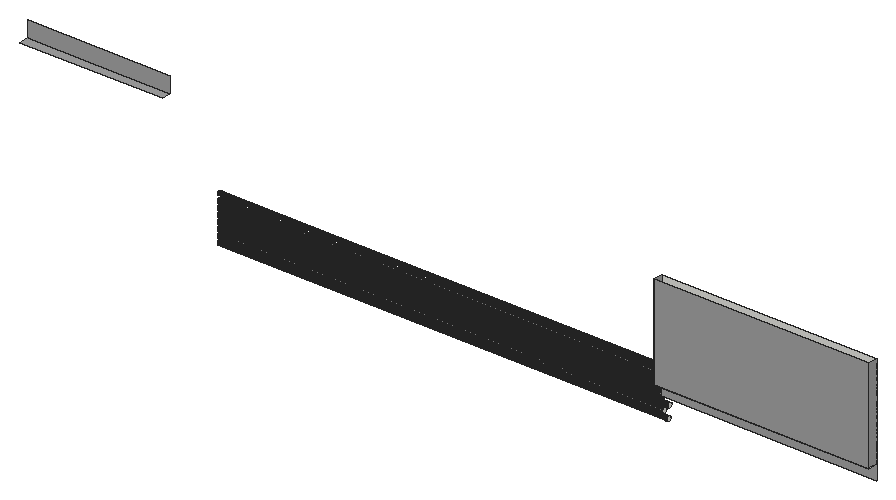
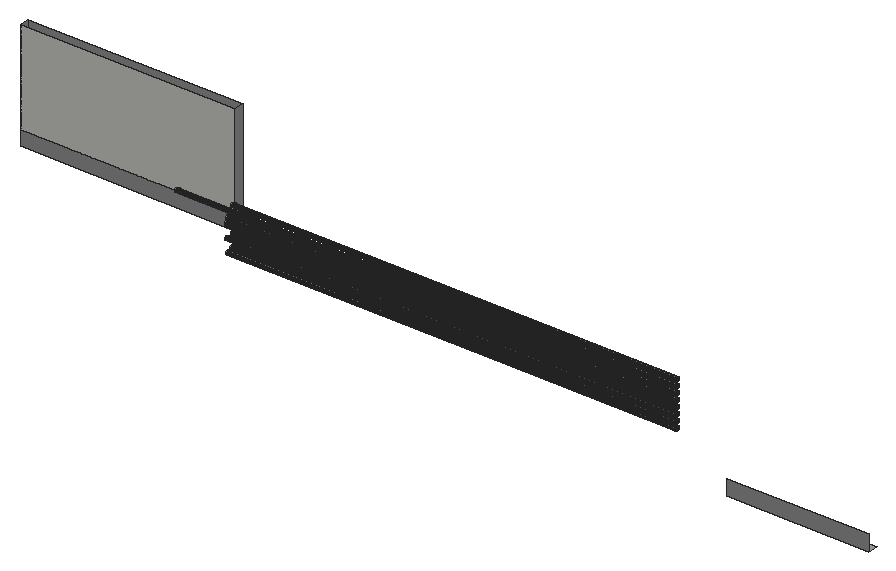
# SketchUp Ruby script. Lengths in inches.
U = 1.inch
M = Sketchup.active_model
def pt(a) = Geom::Point3d.new(a.map { |v| v * U })
def face(e, loops, mat)
  f = e.add_face(loops[0].map { |a| pt(a) })
  loops[1..].each { |l| e.add_face(l.map { |a| pt(a) }).erase! }
  f.material = f.back_material = mat if mat
  f
end
# faces: each face lists its corners as indices into pts; further lists are holes
def faces(e, pts, list, mat = nil) = list.each { |f| face(e, (f[0].is_a?(Array) ? f : [f]).map { |l| l.map { |i| pts[i] } }, mat) }
# xy, xz, yz: faces in a plane at the given z, y or x. An outline is a flat list of corners, or four numbers for a rectangle; further outlines are holes
def ring(l) = l.size == 4 ? [[l[0], l[1]], [l[2], l[1]], [l[2], l[3]], [l[0], l[3]]] : l.each_slice(2).to_a
def flat(e, list, mat, &to3) = list.each { |f| face(e, (f[0].is_a?(Array) ? f : [f]).map { |l| ring(l).map { |u, v| to3.(u, v) } }, mat) }
def xy(e, z, list, mat = nil) = flat(e, list, mat) { |x, y| [x, y, z] }
def xz(e, y, list, mat = nil) = flat(e, list, mat) { |x, z| [x, y, z] }
def yz(e, x, list, mat = nil) = flat(e, list, mat) { |y, z| [x, y, z] }
def lines(e, pts, list) = list.each { |a, b| e.add_line(pt(pts[a]), pt(pts[b])) }
# prism: a flat outline (further loops are holes) pulled along v
def prism(e, loops, v, mat = nil)
  f = face(e, loops, mat); d = Geom::Vector3d.new(v.map { |x| x * U })
  f.pushpull(f.normal.samedirection?(d) ? d.length : -d.length)
end
def box(e, o, s, mat = nil) = prism(e, [[o, [o[0] + s[0], o[1], o[2]], [o[0] + s[0], o[1] + s[1], o[2]], [o[0], o[1] + s[1], o[2]]]], [0, 0, s[2]], mat)
def at(x, y, z, deg = 0) = Geom::Transformation.translation(pt([x, y, z])) * Geom::Transformation.rotation(ORIGIN, Z_AXIS, deg.degrees)
def axes(o, x, y, z) = Geom::Transformation.new([*x, 0, *y, 0, *z, 0, *pt(o).to_a, 1])
def part(name) = M.definitions.add(name)
# library, detail: a bought-in or finely detailed component or shape, given as its bounding box
def library(name, o, s) = part(name).tap { |d| box(d.entities, o, s) }
def detail(e, o, s) = box(e.add_group.entities, o, s)
def put(e, d, t, mat = nil) = e.add_instance(d, t).tap { |i| i.material = mat if mat }
def group(e, t, mat = nil) = e.add_group.tap { |g| g.transformation = t; g.material = mat if mat }.entities
root = M.entities
M.materials.add("[0133_Gray]").color = [128, 128, 128]
M.materials.add("[Pavers Flagstone Gray]").color = [162, 162, 162]
xy(root,165.99,[[229.62,0,297.58,3]],"[Pavers Flagstone Gray]")
xy(root,166.5625,[[0,36,45.0625,39]],"[Pavers Flagstone Gray]")
xz(root,0,[[229.62,165.99,297.58,195.875]],"[Pavers Flagstone Gray]")
xz(root,3,[[229.62,165.99,297.58,195.875]])
xz(root,3,[[229.62,161.3125,297.58,165.99]],"[Pavers Flagstone Gray]")
xz(root,39,[[0,166.5625,45.0625,171.57]],"[Pavers Flagstone Gray]")
yz(root,229.62,[[4.01,168.41,4.17,168.43,4.32,168.49,4.45,168.59,4.55,168.72,4.61,168.87,4.63,169.03,4.61,169.19,4.55,169.34,4.45,169.47,4.32,169.57,4.17,169.64,4.01,169.66,3.84,169.64,3.69,169.57,3.5625,169.47,3.46,169.34,3.4,169.19,3.38,169.03,3.4,168.87,3.46,168.72,3.5625,168.59,3.69,168.49,3.84,168.43]])
yz(root,229.62,[[0,165.99,3,195.875]],"[Pavers Flagstone Gray]")
yz(root,229.78,[[4.01,156.41,4.17,156.43,4.32,156.49,4.45,156.59,4.55,156.72,4.61,156.87,4.63,157.03,4.61,157.19,4.55,157.34,4.45,157.47,4.32,157.57,4.17,157.64,4.01,157.66,3.84,157.64,3.69,157.57,3.5625,157.47,3.46,157.34,3.4,157.19,3.38,157.03,3.4,156.87,3.46,156.72,3.5625,156.59,3.69,156.49,3.84,156.43]])
yz(root,231.1,[[4.01,154.41,4.17,154.43,4.32,154.49,4.45,154.59,4.55,154.72,4.61,154.87,4.63,155.03,4.61,155.19,4.55,155.34,4.45,155.47,4.32,155.57,4.17,155.64,4.01,155.66,3.84,155.64,3.69,155.57,3.5625,155.47,3.46,155.34,3.4,155.19,3.38,155.03,3.4,154.87,3.46,154.72,3.5625,154.59,3.69,154.49,3.84,154.43],[4.01,164.41,4.17,164.43,4.32,164.49,4.45,164.59,4.55,164.72,4.61,164.87,4.63,165.03,4.61,165.19,4.55,165.34,4.45,165.47,4.32,165.57,4.17,165.64,4.01,165.66,3.84,165.64,3.69,165.57,3.5625,165.47,3.46,165.34,3.4,165.19,3.38,165.03,3.4,164.87,3.46,164.72,3.5625,164.59,3.69,164.49,3.84,164.43]])
yz(root,231.41,[[4.01,158.41,4.17,158.43,4.32,158.49,4.45,158.59,4.55,158.72,4.61,158.87,4.63,159.03,4.61,159.19,4.55,159.34,4.45,159.47,4.32,159.57,4.17,159.64,4.01,159.66,3.84,159.64,3.69,159.57,3.5625,159.47,3.46,159.34,3.4,159.19,3.38,159.03,3.4,158.87,3.46,158.72,3.5625,158.59,3.69,158.49,3.84,158.43]])
yz(root,231.6,[[4.01,162.41,4.17,162.43,4.32,162.49,4.45,162.59,4.55,162.72,4.61,162.87,4.63,163.03,4.61,163.19,4.55,163.34,4.45,163.47,4.32,163.57,4.17,163.64,4.01,163.66,3.84,163.64,3.69,163.57,3.5625,163.47,3.46,163.34,3.4,163.19,3.38,163.03,3.4,162.87,3.46,162.72,3.5625,162.59,3.69,162.49,3.84,162.43]])
yz(root,247.41,[[4.01,166.41,4.17,166.43,4.32,166.49,4.45,166.59,4.55,166.72,4.61,166.87,4.63,167.03,4.61,167.19,4.55,167.34,4.45,167.47,4.32,167.57,4.17,167.64,4.01,167.66,3.84,167.64,3.69,167.57,3.5625,167.47,3.46,167.34,3.4,167.19,3.38,167.03,3.4,166.87,3.46,166.72,3.5625,166.59,3.69,166.49,3.84,166.43]])
yz(root,297.58,[[0,165.99,3,166.0625]])
yz(root,297.58,[[0,166.0625,3,195.875]],"[Pavers Flagstone Gray]")
p = [[88.53,3.69,154.49],[88.53,3.84,154.43],[231.1,3.84,154.43],[231.1,3.69,154.49],[88.53,4.01,154.41],[231.1,4.01,154.41],
  [88.53,4.17,154.43],[231.1,4.17,154.43],[88.53,4.32,154.49],[231.1,4.32,154.49],[88.53,3.5625,154.59],[231.1,3.5625,154.59],
  [88.53,4.45,154.59],[231.1,4.45,154.59],[88.53,3.46,154.72],[231.1,3.46,154.72],[88.53,4.55,154.72],[231.1,4.55,154.72],
  [88.53,3.4,154.87],[231.1,3.4,154.87],[88.53,4.61,154.87],[231.1,4.61,154.87],[88.53,3.38,155.03],[231.1,3.38,155.03],
  [88.53,4.63,155.03],[231.1,4.63,155.03],[88.53,3.4,155.19],[231.1,3.4,155.19],[88.53,4.61,155.19],[231.1,4.61,155.19],
  [88.53,3.46,155.34],[231.1,3.46,155.34],[88.53,4.55,155.34],[231.1,4.55,155.34],[88.53,3.5625,155.47],[231.1,3.5625,155.47],
  [88.53,4.45,155.47],[231.1,4.45,155.47],[88.53,3.69,155.57],[231.1,3.69,155.57],[88.53,4.32,155.57],[231.1,4.32,155.57],
  [88.53,3.84,155.64],[231.1,3.84,155.64],[88.53,4.01,155.66],[231.1,4.01,155.66],[88.53,4.17,155.64],[231.1,4.17,155.64],
  [88.53,3.69,156.49],[88.53,3.84,156.43],[229.78,3.84,156.43],[229.78,3.69,156.49],[88.53,4.01,156.41],[229.78,4.01,156.41],
  [88.53,4.17,156.43],[229.78,4.17,156.43],[88.53,4.32,156.49],[229.78,4.32,156.49],[88.53,3.5625,156.59],[229.78,3.5625,156.59],
  [88.53,4.45,156.59],[229.78,4.45,156.59],[88.53,3.46,156.72],[229.78,3.46,156.72],[88.53,4.55,156.72],[229.78,4.55,156.72],
  [88.53,3.4,156.87],[229.78,3.4,156.87],[88.53,4.61,156.87],[229.78,4.61,156.87],[88.53,3.38,157.03],[229.78,3.38,157.03],
  [88.53,4.63,157.03],[229.78,4.63,157.03],[88.53,3.4,157.19],[229.78,3.4,157.19],[88.53,4.61,157.19],[229.78,4.61,157.19],
  [88.53,3.46,157.34],[229.78,3.46,157.34],[88.53,4.55,157.34],[229.78,4.55,157.34],[88.53,3.5625,157.47],[229.78,3.5625,157.47],
  [88.53,4.45,157.47],[229.78,4.45,157.47],[88.53,3.69,157.57],[229.78,3.69,157.57],[88.53,4.32,157.57],[229.78,4.32,157.57],
  [88.53,3.84,157.64],[229.78,3.84,157.64],[88.53,4.01,157.66],[229.78,4.01,157.66],[88.53,4.17,157.64],[229.78,4.17,157.64],
  [88.53,3.69,158.49],[88.53,3.84,158.43],[231.41,3.84,158.43],[231.41,3.69,158.49],[88.53,4.01,158.41],[231.41,4.01,158.41],
  [88.53,4.17,158.43],[231.41,4.17,158.43],[88.53,4.32,158.49],[231.41,4.32,158.49],[88.53,3.5625,158.59],[231.41,3.5625,158.59],
  [88.53,4.45,158.59],[231.41,4.45,158.59],[88.53,3.46,158.72],[231.41,3.46,158.72],[88.53,4.55,158.72],[231.41,4.55,158.72],
  [88.53,3.4,158.87],[231.41,3.4,158.87],[88.53,4.61,158.87],[231.41,4.61,158.87],[88.53,3.38,159.03],[231.41,3.38,159.03],
  [88.53,4.63,159.03],[231.41,4.63,159.03],[88.53,3.4,159.19],[231.41,3.4,159.19],[88.53,4.61,159.19],[231.41,4.61,159.19],
  [88.53,3.46,159.34],[231.41,3.46,159.34],[88.53,4.55,159.34],[231.41,4.55,159.34],[88.53,3.5625,159.47],[231.41,3.5625,159.47],
  [88.53,4.45,159.47],[231.41,4.45,159.47],[88.53,3.69,159.57],[231.41,3.69,159.57],[88.53,4.32,159.57],[231.41,4.32,159.57],
  [88.53,3.84,159.64],[231.41,3.84,159.64],[88.53,4.01,159.66],[231.41,4.01,159.66],[88.53,4.17,159.64],[231.41,4.17,159.64],
  [88.53,3.69,160.49],[88.53,3.84,160.43],[229.62,3.84,160.43],[229.62,3.69,160.49],[88.53,4.01,160.41],[229.62,4.01,160.41],
  [88.53,4.17,160.43],[229.62,4.17,160.43],[88.53,4.32,160.49],[229.62,4.32,160.49],[88.53,3.5625,160.59],[229.62,3.5625,160.59],
  [88.53,4.45,160.59],[229.62,4.45,160.59],[88.53,3.46,160.72],[229.62,3.46,160.72],[88.53,4.55,160.72],[229.62,4.55,160.72],
  [88.53,3.4,160.87],[229.62,3.4,160.87],[88.53,4.61,160.87],[229.62,4.61,160.87],[88.53,3.38,161.03],[229.62,3.38,161.03],
  [88.53,4.63,161.03],[229.62,4.63,161.03],[88.53,3.4,161.19],[229.62,3.4,161.19],[88.53,4.61,161.19],[229.62,4.61,161.19],
  [88.53,3.46,161.34],[229.62,3.46,161.34],[88.53,4.55,161.34],[229.62,4.55,161.34],[88.53,3.5625,161.47],[229.62,3.5625,161.47],
  [88.53,4.45,161.47],[229.62,4.45,161.47],[88.53,3.69,161.57],[229.62,3.69,161.57],[88.53,4.32,161.57],[229.62,4.32,161.57],
  [88.53,3.84,161.64],[229.62,3.84,161.64],[88.53,4.01,161.66],[229.62,4.01,161.66],[88.53,4.17,161.64],[229.62,4.17,161.64],
  [88.53,3.69,162.49],[88.53,3.84,162.43],[231.6,3.84,162.43],[231.6,3.69,162.49],[88.53,4.01,162.41],[231.6,4.01,162.41],
  [88.53,4.17,162.43],[231.6,4.17,162.43],[88.53,4.32,162.49],[231.6,4.32,162.49],[88.53,3.5625,162.59],[231.6,3.5625,162.59],
  [88.53,4.45,162.59],[231.6,4.45,162.59],[88.53,3.46,162.72],[231.6,3.46,162.72],[88.53,4.55,162.72],[231.6,4.55,162.72],
  [88.53,3.4,162.87],[231.6,3.4,162.87],[88.53,4.61,162.87],[231.6,4.61,162.87],[88.53,3.38,163.03],[231.6,3.38,163.03],
  [88.53,4.63,163.03],[231.6,4.63,163.03],[88.53,3.4,163.19],[231.6,3.4,163.19],[88.53,4.61,163.19],[231.6,4.61,163.19],
  [88.53,3.46,163.34],[231.6,3.46,163.34],[88.53,4.55,163.34],[231.6,4.55,163.34],[88.53,3.5625,163.47],[231.6,3.5625,163.47],
  [88.53,4.45,163.47],[231.6,4.45,163.47],[88.53,3.69,163.57],[231.6,3.69,163.57],[88.53,4.32,163.57],[231.6,4.32,163.57],
  [88.53,3.84,163.64],[231.6,3.84,163.64],[88.53,4.01,163.66],[231.6,4.01,163.66],[88.53,4.17,163.64],[231.6,4.17,163.64],
  [88.53,3.69,164.49],[88.53,3.84,164.43],[231.1,3.84,164.43],[231.1,3.69,164.49],[88.53,4.01,164.41],[231.1,4.01,164.41],
  [88.53,4.17,164.43],[231.1,4.17,164.43],[88.53,4.32,164.49],[231.1,4.32,164.49],[88.53,3.5625,164.59],[231.1,3.5625,164.59],
  [88.53,4.45,164.59],[231.1,4.45,164.59],[88.53,3.46,164.72],[231.1,3.46,164.72],[88.53,4.55,164.72],[231.1,4.55,164.72],
  [88.53,3.4,164.87],[231.1,3.4,164.87],[88.53,4.61,164.87],[231.1,4.61,164.87],[88.53,3.38,165.03],[231.1,3.38,165.03],
  [88.53,4.63,165.03],[231.1,4.63,165.03],[88.53,3.4,165.19],[231.1,3.4,165.19],[88.53,4.61,165.19],[231.1,4.61,165.19],
  [88.53,3.46,165.34],[231.1,3.46,165.34],[88.53,4.55,165.34],[231.1,4.55,165.34],[88.53,3.5625,165.47],[231.1,3.5625,165.47],
  [88.53,4.45,165.47],[231.1,4.45,165.47],[88.53,3.69,165.57],[231.1,3.69,165.57],[88.53,4.32,165.57],[231.1,4.32,165.57],
  [88.53,3.84,165.64],[231.1,3.84,165.64],[88.53,4.01,165.66],[231.1,4.01,165.66],[88.53,4.17,165.64],[231.1,4.17,165.64],
  [88.53,3.69,166.49],[88.53,3.84,166.43],[247.41,3.84,166.43],[247.41,3.69,166.49],[88.53,4.01,166.41],[247.41,4.01,166.41],
  [88.53,4.17,166.43],[247.41,4.17,166.43],[88.53,4.32,166.49],[247.41,4.32,166.49],[88.53,3.5625,166.59],[247.41,3.5625,166.59],
  [88.53,4.45,166.59],[247.41,4.45,166.59],[88.53,3.46,166.72],[247.41,3.46,166.72],[88.53,4.55,166.72],[247.41,4.55,166.72],
  [88.53,3.4,166.87],[247.41,3.4,166.87],[88.53,4.61,166.87],[247.41,4.61,166.87],[88.53,3.38,167.03],[247.41,3.38,167.03],
  [88.53,4.63,167.03],[247.41,4.63,167.03],[88.53,3.4,167.19],[247.41,3.4,167.19],[88.53,4.61,167.19],[247.41,4.61,167.19],
  [88.53,3.46,167.34],[247.41,3.46,167.34],[88.53,4.55,167.34],[247.41,4.55,167.34],[88.53,3.5625,167.47],[247.41,3.5625,167.47],
  [88.53,4.45,167.47],[247.41,4.45,167.47],[88.53,3.69,167.57],[247.41,3.69,167.57],[88.53,4.32,167.57],[247.41,4.32,167.57],
  [88.53,3.84,167.64],[247.41,3.84,167.64],[88.53,4.01,167.66],[247.41,4.01,167.66],[88.53,4.17,167.64],[247.41,4.17,167.64],
  [88.53,3.69,168.49],[88.53,3.84,168.43],[229.62,3.84,168.43],[229.62,3.69,168.49],[88.53,4.01,168.41],[229.62,4.01,168.41],
  [88.53,4.17,168.43],[229.62,4.17,168.43],[88.53,4.32,168.49],[229.62,4.32,168.49],[88.53,3.5625,168.59],[229.62,3.5625,168.59],
  [88.53,4.45,168.59],[229.62,4.45,168.59],[88.53,3.46,168.72],[229.62,3.46,168.72],[88.53,4.55,168.72],[229.62,4.55,168.72],
  [88.53,3.4,168.87],[229.62,3.4,168.87],[88.53,4.61,168.87],[229.62,4.61,168.87],[88.53,3.38,169.03],[229.62,3.38,169.03],
  [88.53,4.63,169.03],[229.62,4.63,169.03],[88.53,3.4,169.19],[229.62,3.4,169.19],[88.53,4.61,169.19],[229.62,4.61,169.19],
  [88.53,3.46,169.34],[229.62,3.46,169.34],[88.53,4.55,169.34],[229.62,4.55,169.34],[88.53,3.5625,169.47],[229.62,3.5625,169.47],
  [88.53,4.45,169.47],[229.62,4.45,169.47],[88.53,3.69,169.57],[229.62,3.69,169.57],[88.53,4.32,169.57],[229.62,4.32,169.57],
  [88.53,3.84,169.64],[229.62,3.84,169.64],[88.53,4.01,169.66],[229.62,4.01,169.66],[88.53,4.17,169.64],[229.62,4.17,169.64]]
faces(root,p,[[0,1,2,3],[1,4,5,2],[4,6,7,5],[6,8,9,7],[10,0,3,11],[8,12,13,9],[14,10,11,15],[12,16,17,13],
  [18,14,15,19],[16,20,21,17],[22,18,19,23],[20,24,25,21],[26,22,23,27],[24,28,29,25],[30,26,27,31],[28,32,33,29],
  [34,30,31,35],[32,36,37,33],[38,34,35,39],[36,40,41,37],[42,38,39,43],[44,42,43,45],[46,44,45,47],[40,46,47,41],
  [48,49,50,51],[49,52,53,50],[52,54,55,53],[54,56,57,55],[58,48,51,59],[56,60,61,57],[62,58,59,63],[60,64,65,61],
  [66,62,63,67],[64,68,69,65],[70,66,67,71],[68,72,73,69],[74,70,71,75],[72,76,77,73],[78,74,75,79],[76,80,81,77],
  [82,78,79,83],[80,84,85,81],[86,82,83,87],[84,88,89,85],[90,86,87,91],[92,90,91,93],[94,92,93,95],[88,94,95,89],
  [96,97,98,99],[97,100,101,98],[100,102,103,101],[102,104,105,103],[106,96,99,107],[104,108,109,105],[110,106,107,111],[108,112,113,109],
  [114,110,111,115],[112,116,117,113],[118,114,115,119],[116,120,121,117],[122,118,119,123],[120,124,125,121],[126,122,123,127],[124,128,129,125],
  [130,126,127,131],[128,132,133,129],[134,130,131,135],[132,136,137,133],[138,134,135,139],[140,138,139,141],[142,140,141,143],[136,142,143,137],
  [144,145,146,147],[145,148,149,146],[148,150,151,149],[150,152,153,151],[154,144,147,155],[152,156,157,153],[158,154,155,159],[156,160,161,157],
  [162,158,159,163],[160,164,165,161],[166,162,163,167],[164,168,169,165],[170,166,167,171],[168,172,173,169],[174,170,171,175],[172,176,177,173],
  [178,174,175,179],[176,180,181,177],[182,178,179,183],[180,184,185,181],[186,182,183,187],[188,186,187,189],[190,188,189,191],[184,190,191,185],
  [192,193,194,195],[193,196,197,194],[196,198,199,197],[198,200,201,199],[202,192,195,203],[200,204,205,201],[206,202,203,207],[204,208,209,205],
  [210,206,207,211],[208,212,213,209],[214,210,211,215],[212,216,217,213],[218,214,215,219],[216,220,221,217],[222,218,219,223],[220,224,225,221],
  [226,222,223,227],[224,228,229,225],[230,226,227,231],[228,232,233,229],[234,230,231,235],[236,234,235,237],[238,236,237,239],[232,238,239,233],
  [240,241,242,243],[241,244,245,242],[244,246,247,245],[246,248,249,247],[250,240,243,251],[248,252,253,249],[254,250,251,255],[252,256,257,253],
  [258,254,255,259],[256,260,261,257],[262,258,259,263],[260,264,265,261],[266,262,263,267],[264,268,269,265],[270,266,267,271],[268,272,273,269],
  [274,270,271,275],[272,276,277,273],[278,274,275,279],[276,280,281,277],[282,278,279,283],[284,282,283,285],[286,284,285,287],[280,286,287,281],
  [288,289,290,291],[289,292,293,290],[292,294,295,293],[294,296,297,295],[298,288,291,299],[296,300,301,297],[302,298,299,303],[300,304,305,301],
  [306,302,303,307],[304,308,309,305],[310,306,307,311],[308,312,313,309],[314,310,311,315],[312,316,317,313],[318,314,315,319],[316,320,321,317],
  [322,318,319,323],[320,324,325,321],[326,322,323,327],[324,328,329,325],[330,326,327,331],[332,330,331,333],[334,332,333,335],[328,334,335,329],
  [336,337,338,339],[337,340,341,338],[340,342,343,341],[342,344,345,343],[346,336,339,347],[344,348,349,345],[350,346,347,351],[348,352,353,349],
  [354,350,351,355],[352,356,357,353],[358,354,355,359],[356,360,361,357],[362,358,359,363],[360,364,365,361],[366,362,363,367],[364,368,369,365],
  [370,366,367,371],[368,372,373,369],[374,370,371,375],[372,376,377,373],[378,374,375,379],[380,378,379,381],[382,380,381,383],[376,382,383,377]],"[0133_Gray]")
